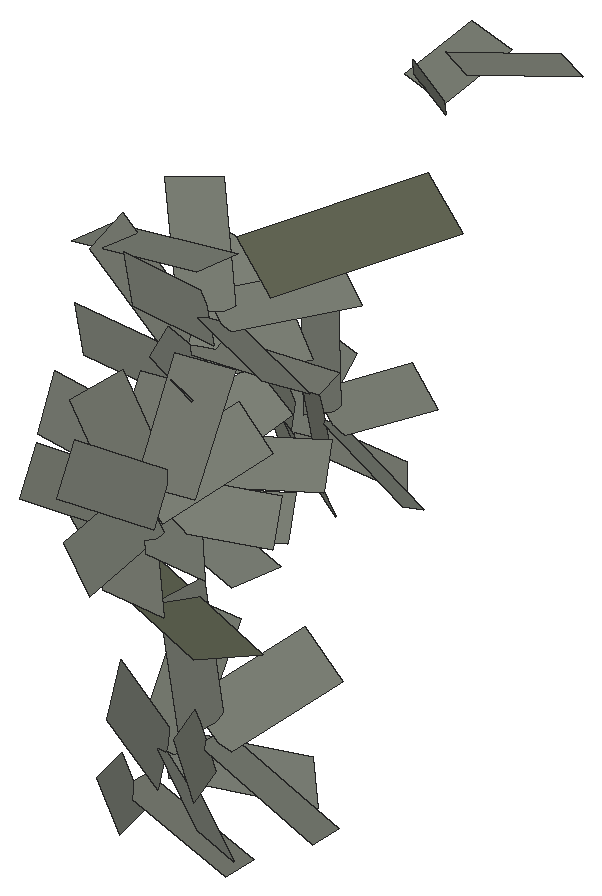
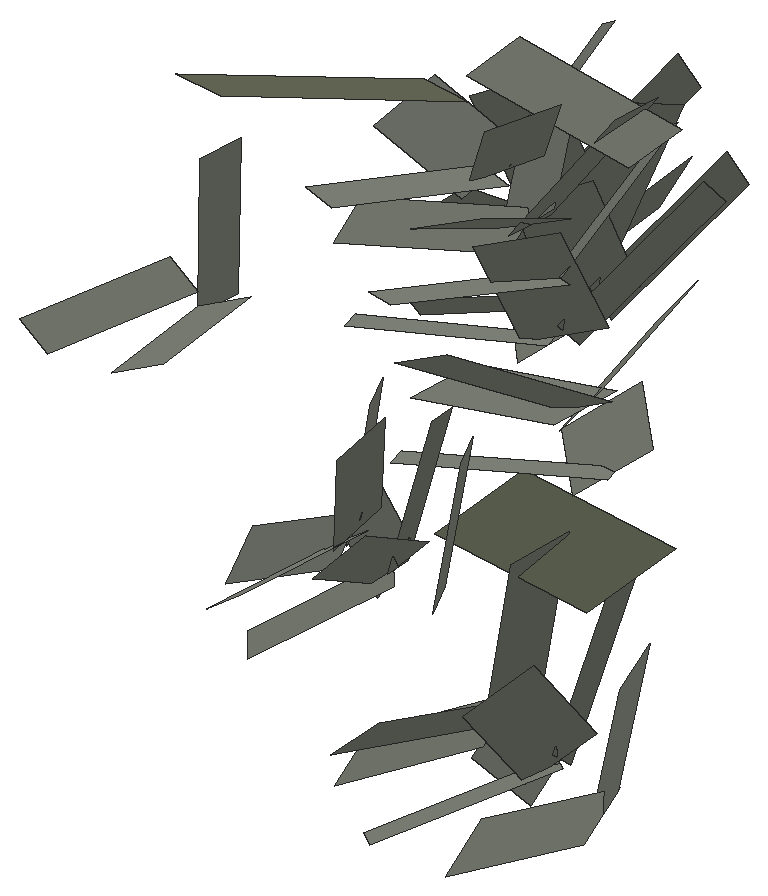
# SketchUp Ruby script. Lengths in inches.
U = 1.inch
M = Sketchup.active_model
def pt(a) = Geom::Point3d.new(a.map { |v| v * U })
def face(e, loops, mat)
  f = e.add_face(loops[0].map { |a| pt(a) })
  loops[1..].each { |l| e.add_face(l.map { |a| pt(a) }).erase! }
  f.material = f.back_material = mat if mat
  f
end
# faces: each face lists its corners as indices into pts; further lists are holes
def faces(e, pts, list, mat = nil) = list.each { |f| face(e, (f[0].is_a?(Array) ? f : [f]).map { |l| l.map { |i| pts[i] } }, mat) }
# xy, xz, yz: faces in a plane at the given z, y or x. An outline is a flat list of corners, or four numbers for a rectangle; further outlines are holes
def ring(l) = l.size == 4 ? [[l[0], l[1]], [l[2], l[1]], [l[2], l[3]], [l[0], l[3]]] : l.each_slice(2).to_a
def flat(e, list, mat, &to3) = list.each { |f| face(e, (f[0].is_a?(Array) ? f : [f]).map { |l| ring(l).map { |u, v| to3.(u, v) } }, mat) }
def xy(e, z, list, mat = nil) = flat(e, list, mat) { |x, y| [x, y, z] }
def xz(e, y, list, mat = nil) = flat(e, list, mat) { |x, z| [x, y, z] }
def yz(e, x, list, mat = nil) = flat(e, list, mat) { |y, z| [x, y, z] }
def lines(e, pts, list) = list.each { |a, b| e.add_line(pt(pts[a]), pt(pts[b])) }
# prism: a flat outline (further loops are holes) pulled along v
def prism(e, loops, v, mat = nil)
  f = face(e, loops, mat); d = Geom::Vector3d.new(v.map { |x| x * U })
  f.pushpull(f.normal.samedirection?(d) ? d.length : -d.length)
end
def box(e, o, s, mat = nil) = prism(e, [[o, [o[0] + s[0], o[1], o[2]], [o[0] + s[0], o[1] + s[1], o[2]], [o[0], o[1] + s[1], o[2]]]], [0, 0, s[2]], mat)
def at(x, y, z, deg = 0) = Geom::Transformation.translation(pt([x, y, z])) * Geom::Transformation.rotation(ORIGIN, Z_AXIS, deg.degrees)
def axes(o, x, y, z) = Geom::Transformation.new([*x, 0, *y, 0, *z, 0, *pt(o).to_a, 1])
def part(name) = M.definitions.add(name)
# library, detail: a bought-in or finely detailed component or shape, given as its bounding box
def library(name, o, s) = part(name).tap { |d| box(d.entities, o, s) }
def detail(e, o, s) = box(e.add_group.entities, o, s)
def put(e, d, t, mat = nil) = e.add_instance(d, t).tap { |i| i.material = mat if mat }
def group(e, t, mat = nil) = e.add_group.tap { |g| g.transformation = t; g.material = mat if mat }.entities
root = M.entities
M.materials.add("viburnumblaasdfas0df1w06d").color = [98, 102, 84]
M.materials.add("viburnumbladsadfasdfad0w122").color = [125, 129, 119]
c1 = part("Component\#315")
p = [[0.25,0,0],[2.05,0.01,0.35],[1.81,4.2,1.66],[0,4.19,1.3125]]
faces(c1.entities,p,[[0,1,2,3]],"viburnumbladsadfasdfad0w122")
c2 = part("viburnumblad2")
put(c2.entities,c1,axes([-19.23,-4.49,-32.18],[83.35428,0,0],[0,79.38502,0],[0,0,83.35428]))
c3 = part("Component\#314")
p = [[0.14,0,0],[2.58,0.05,0.25],[2.44,5.11,2.64],[0,5.05,2.39]]
faces(c3.entities,p,[[0,1,2,3]],"viburnumblaasdfas0df1w06d")
c4 = part("viburnumblad1\#2")
put(c4.entities,c3,axes([-37.25,6.23,19.31],[75.98784,0,0],[0,65.50676,0],[0,0,75.98784]))
put(root,c2,axes([1241.48,293.02,20.39],[0.00435,0.00477,-0.00798],[-0.00392,0.00825,0.00263],[0.00812,0.00193,0.0048]))
put(root,c2,axes([1241.43,292.96,18.53],[-0.0065,0.00265,0.00695],[0.00166,-0.0098,0.00501],[0.00741,0.00415,0.00458]))
put(root,c2,axes([1243,286.66,25.51],[-0.00283,0.01146,0.00038],[-0.0094,-0.00257,0.00741],[0.00704,0.00146,0.00821]))
put(root,c2,axes([1242.28,292.78,19.51],[-0.00523,0.00868,0.00226],[-0.00357,-0.00459,0.00897],[0.00802,0.00357,0.00411]))
put(root,c2,axes([1242.72,287.04,24.1],[-0.00853,0.00601,0.00433],[-0.00446,-0.01051,0.00545],[0.00645,0.00235,0.00846]))
put(root,c2,axes([1241.88,286.62,12.66],[0.00427,0.00859,-0.00811],[-0.005,0.00913,0.00703],[0.0107,0.00084,0.00653]))
put(root,c2,axes([1243.16,285.38,21.67],[-0.00501,0.0098,0.00679],[-0.00808,-0.00821,0.00589],[0.00877,-0.00196,0.0093]))
put(root,c2,axes([1239.68,287.91,28.49],[-0.00073,-0.01199,-0.00108],[0.01339,-0.00063,-0.00213],[0.0019,-0.00123,0.01236]))
put(root,c2,axes([1241.72,299.01,29.15],[0.00769,0.00057,-0.00539],[-0.00261,0.00972,-0.00258],[0.00555,0.0035,0.00706]))
put(root,c2,axes([1241.86,286.96,10.17],[-0.00779,-0.00011,0.00854],[0.00262,-0.01208,0.00224],[0.0089,0.00345,0.00816]))
put(root,c2,axes([1242.76,286.61,20.15],[-0.00997,0.00134,0.00814],[-0.00176,-0.01174,-0.00023],[0.00802,-0.0014,0.01005]))
put(root,c2,axes([1242.82,293.04,20.79],[-0.00062,0.00952,-0.00405],[-0.0058,0.00311,0.00781],[0.00831,0.00266,0.0042]))
put(root,c2,axes([1241.98,285.8125,22.71],[0.00909,0.00791,-0.00471],[-0.00403,0.00937,0.00796],[0.00828,-0.00412,0.00905]))
put(root,c2,axes([1243,286.89,27.11],[0.00489,0.00995,-0.00397],[-0.0081,0.00635,0.00558],[0.00694,0.00038,0.0084]))
put(root,c2,axes([1241.78,287.38,19.18],[-0.00949,-0.00826,0.00492],[0.00532,-0.00908,-0.00498],[0.00706,-0.00173,0.0107]))
put(root,c2,axes([1242.85,286.35,11.4],[-0.00627,0.00896,0.00619],[-0.00305,-0.00837,0.00903],[0.01046,0.00298,0.00629]))
put(root,c2,axes([1241.9,287.3,26.07],[0.00974,0.00261,-0.006],[-0.00192,0.01057,0.00135],[0.0062,-0.00026,0.0089]))
put(root,c4,axes([1239.6,288.64,17],[-0.00406,-0.01328,0.00293],[0.01275,-0.00581,-0.00863],[0.008,0.00014,0.01172]))
put(root,c2,axes([1241.04,286.88,21.625],[0.00997,-0.00134,-0.00814],[0.0038,0.01207,0.00267],[0.00731,-0.00445,0.00969]))
put(root,c2,axes([1243.68,283.6,21.22],[-0.00309,0.00736,0.0079],[-0.00654,-0.00921,0.0057],[0.00929,-0.00262,0.00521]))
put(root,c2,axes([1240.52,287.7,20.19],[0.00481,-0.00941,-0.00652],[0.01076,0.00809,-0.00374],[0.00656,-0.00389,0.01045]))
put(root,c2,axes([1243.54,286.48,13.17],[-0.00141,0.01241,-0.00136],[-0.00618,0.00049,0.01093],[0.01085,0.0019,0.00605]))
put(root,c2,axes([1241.17,288.01,10.67],[0.00148,-0.01296,0.00142],[0.00776,-0.00002,-0.00823],[0.00903,0.00196,0.00851]))
put(root,c2,axes([1241.42,294.37,19.83],[0.00523,-0.00868,-0.00226],[0.00529,0.00516,-0.00737],[0.00696,0.00241,0.00605]))
put(root,c2,axes([1241.34,288.1,24.93],[0.00761,-0.00572,-0.00506],[0.00557,0.01001,-0.00285],[0.00619,-0.00075,0.00889]))
put(root,c2,axes([1242.26,294.22,20.9],[0.00677,-0.00276,-0.00724],[0.0003,0.00981,-0.00339],[0.00756,0.00183,0.00557]))
put(root,c2,axes([1244.27,286.97,26.35],[-0.00889,0.00626,0.00451],[-0.00413,-0.00973,0.00504],[0.00645,0.00235,0.00846]))
put(root,c2,axes([1242.29,293.83,18.99],[-0.00435,-0.00477,0.00798],[0.00611,-0.00825,-0.00162],[0.00685,0.00405,0.00535]))
put(root,c2,axes([1242.8125,283.67,22.42],[0.00746,0.0085,-0.0048],[-0.00195,0.00645,0.00799],[0.00881,-0.00455,0.00477]))
put(root,c2,axes([1243.14,299.1,28.26],[-0.00855,-0.00095,0.00486],[0.00394,-0.00929,0.00471],[0.00385,0.00566,0.0068]))
put(root,c2,axes([1241.77,288.01,12.4],[0.00627,-0.00896,-0.00619],[0.00573,0.0092,-0.00751],[0.00942,0.00088,0.00827]))
put(root,c2,axes([1243.47,293.45,19.75],[-0.00677,0.00276,0.00724],[0.00154,-0.00908,0.00464],[0.00741,0.00415,0.00458]))
put(root,c2,axes([1242.85,287.78,13.76],[0.00745,-0.00026,-0.01011],[-0.00018,0.01255,-0.00046],[0.01011,0.00042,0.00745]))
put(root,c2,axes([1244.22,282.77,22.33],[0.00278,0.01118,0.00257],[-0.00655,-0.00082,0.0102],[0.00931,-0.00357,0.00467]))
put(root,c2,axes([1242.27,300.17,29.58],[0.00853,-0.00582,-0.00111],[0.00461,0.00781,-0.00517],[0.00374,0.00366,0.00797]))
put(root,c2,axes([1243.64,287.72,25.04],[-0.00974,-0.00261,0.006],[0.00353,-0.01123,0.00072],[0.00551,0.00254,0.00899]))
put(root,c2,axes([1242.62,288.09,11.1875],[-0.00427,-0.00859,0.00811],[0.00683,-0.00794,-0.00482],[0.00917,0.00302,0.00803]))
put(root,c2,axes([1242.1,287.68,21.01],[-0.00288,-0.01252,-0.00147],[0.01138,-0.00177,-0.00721],[0.00645,-0.00276,0.01087]))
put(root,c2,axes([1243.73,286.91,21.68],[-0.00909,-0.00791,0.00471],[0.00591,-0.01009,-0.00553],[0.00706,-0.00173,0.0107]))
put(root,c2,axes([1242.92,294.63,19.86],[0.00062,-0.00952,0.00405],[0.00764,-0.00238,-0.00656],[0.00666,0.00333,0.00596]))
put(root,c2,axes([1244.2,287.36,12.02],[-0.00745,0.00026,0.01011],[0.00262,-0.01208,0.00224],[0.00977,0.00344,0.00711]))
put(root,c2,axes([1242.85,288.37,27.03],[0.00889,-0.00626,-0.00451],[0.00557,0.01001,-0.00285],[0.00526,-0.00007,0.00943]))
put(root,c2,axes([1245.08,283.61,21.75],[-0.00733,-0.00034,0.00907],[-0.00172,-0.01154,-0.00184],[0.00876,-0.00225,0.00608]))
put(root,c2,axes([1242.61,288.7,25.53],[0.00283,-0.01146,-0.00038],[0.01049,0.00275,-0.00491],[0.00467,0.00082,0.00968]))
put(root,c2,axes([1242.55,287.34,22.72],[0.00501,-0.0098,-0.00679],[0.00996,0.00749,-0.00346],[0.00656,-0.00389,0.01045]))
put(root,c2,axes([1245.71,282.35,22.61],[-0.00322,0.00766,0.00823],[-0.00606,-0.00853,0.00527],[0.00929,-0.00262,0.00521]))
put(root,c2,axes([1243.27,284.84,22.62],[0.0022,-0.00655,-0.00816],[0.00813,0.00764,-0.00386],[0.00785,-0.0054,0.00541]))
put(root,c2,axes([1243.77,283.6,23.34],[0.00733,0.00034,-0.00907],[0.00348,0.00978,0.00299],[0.00808,-0.00497,0.00546]))
put(root,c2,axes([1244.86,282.55,23.79],[0.00715,0.00814,-0.0046],[-0.00216,0.00716,0.00888],[0.00881,-0.00455,0.00477]))
put(root,c2,axes([1243.51,288.66,12.62],[0.00141,-0.01241,0.00136],[0.00862,-0.00002,-0.00914],[0.00903,0.00196,0.00851]))
put(root,c2,axes([1244.125,288.45,26.27],[-0.00489,-0.00995,0.00397],[0.00954,-0.00607,-0.00338],[0.00477,0.0019,0.00949]))
put(root,c4,axes([1243.68,288.41,28.38],[0.01127,-0.00662,-0.00498],[0.00702,0.01432,-0.0031],[0.00548,-0.00011,0.01154]))
